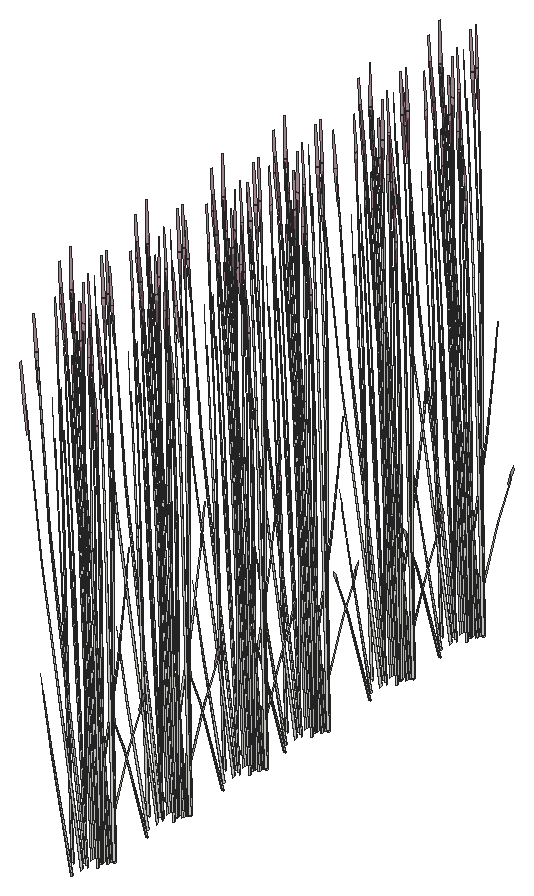
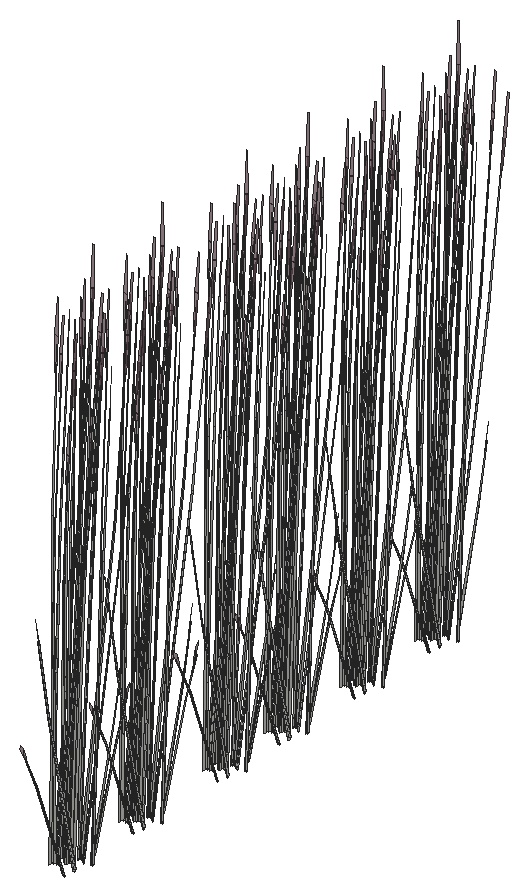
# SketchUp Ruby script. Lengths in inches.
U = 1.inch
M = Sketchup.active_model
def pt(a) = Geom::Point3d.new(a.map { |v| v * U })
def face(e, loops, mat)
  f = e.add_face(loops[0].map { |a| pt(a) })
  loops[1..].each { |l| e.add_face(l.map { |a| pt(a) }).erase! }
  f.material = f.back_material = mat if mat
  f
end
# faces: each face lists its corners as indices into pts; further lists are holes
def faces(e, pts, list, mat = nil) = list.each { |f| face(e, (f[0].is_a?(Array) ? f : [f]).map { |l| l.map { |i| pts[i] } }, mat) }
# xy, xz, yz: faces in a plane at the given z, y or x. An outline is a flat list of corners, or four numbers for a rectangle; further outlines are holes
def ring(l) = l.size == 4 ? [[l[0], l[1]], [l[2], l[1]], [l[2], l[3]], [l[0], l[3]]] : l.each_slice(2).to_a
def flat(e, list, mat, &to3) = list.each { |f| face(e, (f[0].is_a?(Array) ? f : [f]).map { |l| ring(l).map { |u, v| to3.(u, v) } }, mat) }
def xy(e, z, list, mat = nil) = flat(e, list, mat) { |x, y| [x, y, z] }
def xz(e, y, list, mat = nil) = flat(e, list, mat) { |x, z| [x, y, z] }
def yz(e, x, list, mat = nil) = flat(e, list, mat) { |y, z| [x, y, z] }
def lines(e, pts, list) = list.each { |a, b| e.add_line(pt(pts[a]), pt(pts[b])) }
# prism: a flat outline (further loops are holes) pulled along v
def prism(e, loops, v, mat = nil)
  f = face(e, loops, mat); d = Geom::Vector3d.new(v.map { |x| x * U })
  f.pushpull(f.normal.samedirection?(d) ? d.length : -d.length)
end
def box(e, o, s, mat = nil) = prism(e, [[o, [o[0] + s[0], o[1], o[2]], [o[0] + s[0], o[1] + s[1], o[2]], [o[0], o[1] + s[1], o[2]]]], [0, 0, s[2]], mat)
def at(x, y, z, deg = 0) = Geom::Transformation.translation(pt([x, y, z])) * Geom::Transformation.rotation(ORIGIN, Z_AXIS, deg.degrees)
def axes(o, x, y, z) = Geom::Transformation.new([*x, 0, *y, 0, *z, 0, *pt(o).to_a, 1])
def part(name) = M.definitions.add(name)
# library, detail: a bought-in or finely detailed component or shape, given as its bounding box
def library(name, o, s) = part(name).tap { |d| box(d.entities, o, s) }
def detail(e, o, s) = box(e.add_group.entities, o, s)
def put(e, d, t, mat = nil) = e.add_instance(d, t).tap { |i| i.material = mat if mat }
def group(e, t, mat = nil) = e.add_group.tap { |g| g.transformation = t; g.material = mat if mat }.entities
root = M.entities
M.materials.add("LightPink_Translucent").color = [144, 107, 117]
M.materials["LightPink_Translucent"].alpha = 0.75
c1 = part("blade")
p = [[2.15,0.21,22],[0,0.17,0],[0.09,0.45,0],[2.18,0.31,22],[2.29,0.31,22],[0.38,0.45,0],
  [2.48,0.24,33],[2.49,0.24,33],[2.48,0.22,33]]
faces(c1.entities,p,[[0,1,2,3],[4,5,2,3],[6,3,4,7],[8,0,3,6]])
c2 = part("seeds")
p = [[0.3,-0.1,1.38],[-0.01,-0.03,1.59],[-0.01,-0.03,0.03],[0.14,-0.07,-0.07],[0.29,-0.03,3],[0.15,0.01,3.11]]
faces(c2.entities,p,[[0,1,2,3],[1,0,4,5]],"LightPink_Translucent")
c3 = part("blade with seeds")
put(c3.entities,c1,at(0,0,0))
put(c3.entities,c2,axes([2.4,0.25,30.99],[1.5799,-0.05474,1.17369],[-0.12525,1.92788,0.29478],[-0.07173,-0.02425,1.56792]))
put(root,c3,axes([333,451.01,49.85],[-0.20736,-0.4007,-0.61707],[0.59731,-0.14431,-0.16195],[-0.02292,-0.13569,1.36206]))
put(root,c3,axes([333.61,449.38,49.88],[-0.34892,0.22417,-0.0344],[-0.3197,-0.24551,-0.15595],[-0.02251,-0.06957,0.51438]))
put(root,c3,axes([333.32,451.11,49.95],[0.24498,-0.3521,-0.39531],[0.50902,0.16945,0.19025],[0,-0.08116,1.26923]))
put(root,c3,axes([332.02,450.96,49.79],[0.35245,-0.2438,-0.27372],[0.35245,0.2438,0.27372],[0,-0.07853,1.22797]))
put(root,c3,axes([333.25,451.4,50.36],[-0.56863,-0.18645,-0.25709],[0.2738,-0.39352,-0.44182],[-0.01787,-0.09662,1.41118]))
put(root,c3,axes([332.02,451.3125,50.19],[0,0.39075,0.43871],[-0.56491,0,0],[0,-0.089,1.3917]))
put(root,c3,axes([333.42,451.17,50.09],[0.21952,0.43694,0.40429],[-0.62724,0.15194,0.15865],[0.00767,-0.08029,1.40366]))
put(root,c3,axes([333.31,451.51,50.4],[-0.24498,0.3521,0.39531],[-0.50902,-0.16945,-0.19025],[0,-0.08116,1.26923]))
put(root,c3,axes([334.36,451.55,50.03],[-0.46965,-0.33633,-0.05417],[0.46994,-0.33653,0],[-0.0164,-0.01174,1.55135]))
put(root,c3,axes([333.47,451.59,50.09],[0.63817,0.08233,0.40429],[-0.12987,0.46497,0.15865],[-0.09326,-0.0449,1.40366]))
put(root,c3,axes([333.13,452.34,50.1875],[0.54257,-0.10371,0.15589],[0.13397,0.38597,0.31002],[-0.04839,-0.05624,1.41735]))
put(root,c3,axes([333.94,452.25,49.95],[-0.16474,-0.33688,0],[0.47043,-0.11798,0],[0,0,1.36402]))
put(root,c3,axes([334.74,452.36,50.1875],[0.14586,-0.38834,0.15589],[0.53375,0.1099,0.31002],[-0.0922,0.00189,1.41735]))
put(root,c3,axes([333.83,452.4,49.94],[-0.50902,-0.17543,0],[0.24498,-0.36452,0],[0,0,1.43768]))
put(root,c3,axes([334.49,451.67,50.4],[0.54829,-0.02412,0.39531],[0.04958,0.40041,-0.19025],[-0.09816,0.04058,1.26923]))
put(root,c3,axes([334.61,452.79,49.9375],[-0.31175,-0.39292,-0.04544],[0.52815,-0.21836,0.456],[-0.13015,0.03741,1.44584]))
put(root,c3,axes([334.5,451.84,50.3125],[0.37303,0.23477,0.12794],[-0.31115,0.26487,-0.36534],[-0.08661,0.03581,1.11991]))
put(root,c3,axes([334.89,452.57,50.19],[0.47255,-0.19538,0.43871],[0.28245,0.35034,0],[-0.10763,0.0445,1.3917]))
put(root,c3,axes([334.46,452.74,49.79],[-0.47106,-0.09668,-0.27372],[0.11861,-0.34048,0.27372],[-0.09497,0.03926,1.22797]))
put(root,c3,axes([334.38,451.76,50.36],[0.05884,0.44587,-0.25709],[-0.6128,0.02696,-0.44182],[-0.10791,0.05939,1.41118]))
put(root,c3,axes([334.62,452.59,50.06],[0.63212,0.12701,0.27176],[-0.15814,0.45398,-0.32244],[-0.10462,0.05682,1.45692]))
put(root,c3,axes([335,452.84,50.1],[0.31568,0.39156,0],[-0.52815,0.21836,-0.456],[-0.12029,0.04973,1.44655]))
put(root,c3,axes([333.34,452.96,49.32],[0.08172,-0.02126,1.55816],[0.49154,0.11703,-0.23804],[0.01437,0.1319,0.26541]))
put(root,c3,axes([332.21,453.01,50.49],[0.45869,-0.0692,0.0575],[0.10545,0.27878,-0.76259],[-0.02908,0.14112,0.68355]))
put(root,c3,axes([333.7,458.625,49.32],[-0.08469,0.01408,1.55816],[-0.46834,-0.15847,-0.23804],[0.00786,-0.13218,0.26541]))
put(root,c3,axes([333,460.52,49.85],[-0.20736,-0.4007,-0.61707],[0.59731,-0.14431,-0.16195],[-0.02292,-0.13569,1.36206]))
put(root,c3,axes([333.61,458.9,49.88],[-0.34892,0.22417,-0.0344],[-0.3197,-0.24551,-0.15595],[-0.02251,-0.06957,0.51438]))
put(root,c3,axes([333.32,460.625,49.95],[0.24498,-0.3521,-0.39531],[0.50902,0.16945,0.19025],[0,-0.08116,1.26923]))
put(root,c3,axes([332.02,460.47,49.79],[0.35245,-0.2438,-0.27372],[0.35245,0.2438,0.27372],[0,-0.07853,1.22797]))
put(root,c3,axes([333.25,460.92,50.36],[-0.56863,-0.18645,-0.25709],[0.2738,-0.39352,-0.44182],[-0.01787,-0.09662,1.41118]))
put(root,c3,axes([332.02,460.83,50.19],[0,0.39075,0.43871],[-0.56491,0,0],[0,-0.089,1.3917]))
put(root,c3,axes([333.42,460.68,50.09],[0.21952,0.43694,0.40429],[-0.62724,0.15194,0.15865],[0.00767,-0.08029,1.40366]))
put(root,c3,axes([333.31,461.02,50.4],[-0.24498,0.3521,0.39531],[-0.50902,-0.16945,-0.19025],[0,-0.08116,1.26923]))
put(root,c3,axes([334.36,461.07,50.03],[-0.46965,-0.33633,-0.05417],[0.46994,-0.33653,0],[-0.0164,-0.01174,1.55135]))
put(root,c3,axes([333.47,461.11,50.09],[0.63817,0.08233,0.40429],[-0.12987,0.46497,0.15865],[-0.09326,-0.0449,1.40366]))
put(root,c3,axes([333.13,461.85,50.1875],[0.54257,-0.10371,0.15589],[0.13397,0.38597,0.31002],[-0.04839,-0.05624,1.41735]))
put(root,c3,axes([333.94,461.76,49.95],[-0.16474,-0.33688,0],[0.47043,-0.11798,0],[0,0,1.36402]))
put(root,c3,axes([334.74,461.87,50.1875],[0.14586,-0.38834,0.15589],[0.53375,0.1099,0.31002],[-0.0922,0.00189,1.41735]))
put(root,c3,axes([333.83,461.91,49.94],[-0.50902,-0.17543,0],[0.24498,-0.36452,0],[0,0,1.43768]))
put(root,c3,axes([334.49,461.19,50.4],[0.54829,-0.02412,0.39531],[0.04958,0.40041,-0.19025],[-0.09816,0.04058,1.26923]))
put(root,c3,axes([334.61,462.31,49.9375],[-0.31175,-0.39292,-0.04544],[0.52815,-0.21836,0.456],[-0.13015,0.03741,1.44584]))
put(root,c3,axes([334.5,461.36,50.3125],[0.37303,0.23477,0.12794],[-0.31115,0.26487,-0.36534],[-0.08661,0.03581,1.11991]))
put(root,c3,axes([334.89,462.08,50.19],[0.47255,-0.19538,0.43871],[0.28245,0.35034,0],[-0.10763,0.0445,1.3917]))
put(root,c3,axes([334.46,462.26,49.79],[-0.47106,-0.09668,-0.27372],[0.11861,-0.34048,0.27372],[-0.09497,0.03926,1.22797]))
put(root,c3,axes([334.38,461.27,50.36],[0.05884,0.44587,-0.25709],[-0.6128,0.02696,-0.44182],[-0.10791,0.05939,1.41118]))
put(root,c3,axes([334.62,462.11,50.06],[0.63212,0.12701,0.27176],[-0.15814,0.45398,-0.32244],[-0.10462,0.05682,1.45692]))
put(root,c3,axes([335,462.35,50.1],[0.31568,0.39156,0],[-0.52815,0.21836,-0.456],[-0.12029,0.04973,1.44655]))
put(root,c3,axes([333.34,462.47,49.32],[0.08172,-0.02126,1.55816],[0.49154,0.11703,-0.23804],[0.01437,0.1319,0.26541]))
put(root,c3,axes([332.21,462.52,50.49],[0.45869,-0.0692,0.0575],[0.10545,0.27878,-0.76259],[-0.02908,0.14112,0.68355]))
put(root,c3,axes([333.7,468.18,49.32],[-0.08469,0.01408,1.55816],[-0.46834,-0.15847,-0.23804],[0.00786,-0.13218,0.26541]))
put(root,c3,axes([333,470.08,49.85],[-0.20736,-0.4007,-0.61707],[0.59731,-0.14431,-0.16195],[-0.02292,-0.13569,1.36206]))
put(root,c3,axes([333.61,468.45,49.88],[-0.34892,0.22417,-0.0344],[-0.3197,-0.24551,-0.15595],[-0.02251,-0.06957,0.51438]))
put(root,c3,axes([333.32,470.18,49.95],[0.24498,-0.3521,-0.39531],[0.50902,0.16945,0.19025],[0,-0.08116,1.26923]))
put(root,c3,axes([332.02,470.03,49.79],[0.35245,-0.2438,-0.27372],[0.35245,0.2438,0.27372],[0,-0.07853,1.22797]))
put(root,c3,axes([333.25,470.47,50.36],[-0.56863,-0.18645,-0.25709],[0.2738,-0.39352,-0.44182],[-0.01787,-0.09662,1.41118]))
put(root,c3,axes([332.02,470.38,50.19],[0,0.39075,0.43871],[-0.56491,0,0],[0,-0.089,1.3917]))
put(root,c3,axes([333.42,470.24,50.09],[0.21952,0.43694,0.40429],[-0.62724,0.15194,0.15865],[0.00767,-0.08029,1.40366]))
put(root,c3,axes([333.31,470.58,50.4],[-0.24498,0.3521,0.39531],[-0.50902,-0.16945,-0.19025],[0,-0.08116,1.26923]))
put(root,c3,axes([334.36,470.625,50.03],[-0.46965,-0.33633,-0.05417],[0.46994,-0.33653,0],[-0.0164,-0.01174,1.55135]))
put(root,c3,axes([333.47,470.66,50.09],[0.63817,0.08233,0.40429],[-0.12987,0.46497,0.15865],[-0.09326,-0.0449,1.40366]))
put(root,c3,axes([333.13,471.41,50.1875],[0.54257,-0.10371,0.15589],[0.13397,0.38597,0.31002],[-0.04839,-0.05624,1.41735]))
put(root,c3,axes([333.94,471.32,49.95],[-0.16474,-0.33688,0],[0.47043,-0.11798,0],[0,0,1.36402]))
put(root,c3,axes([334.74,471.43,50.1875],[0.14586,-0.38834,0.15589],[0.53375,0.1099,0.31002],[-0.0922,0.00189,1.41735]))
put(root,c3,axes([333.83,471.47,49.94],[-0.50902,-0.17543,0],[0.24498,-0.36452,0],[0,0,1.43768]))
put(root,c3,axes([334.49,470.74,50.4],[0.54829,-0.02412,0.39531],[0.04958,0.40041,-0.19025],[-0.09816,0.04058,1.26923]))
put(root,c3,axes([334.61,471.86,49.9375],[-0.31175,-0.39292,-0.04544],[0.52815,-0.21836,0.456],[-0.13015,0.03741,1.44584]))
put(root,c3,axes([334.5,470.91,50.3125],[0.37303,0.23477,0.12794],[-0.31115,0.26487,-0.36534],[-0.08661,0.03581,1.11991]))
put(root,c3,axes([334.89,471.64,50.19],[0.47255,-0.19538,0.43871],[0.28245,0.35034,0],[-0.10763,0.0445,1.3917]))
put(root,c3,axes([334.46,471.8125,49.79],[-0.47106,-0.09668,-0.27372],[0.11861,-0.34048,0.27372],[-0.09497,0.03926,1.22797]))
put(root,c3,axes([334.38,470.83,50.36],[0.05884,0.44587,-0.25709],[-0.6128,0.02696,-0.44182],[-0.10791,0.05939,1.41118]))
put(root,c3,axes([334.62,471.66,50.06],[0.63212,0.12701,0.27176],[-0.15814,0.45398,-0.32244],[-0.10462,0.05682,1.45692]))
put(root,c3,axes([335,471.91,50.1],[0.31568,0.39156,0],[-0.52815,0.21836,-0.456],[-0.12029,0.04973,1.44655]))
put(root,c3,axes([333.7,475.98,49.32],[-0.08469,0.01408,1.55816],[-0.46834,-0.15847,-0.23804],[0.00786,-0.13218,0.26541]))
put(root,c3,axes([333.34,472.03,49.32],[0.08172,-0.02126,1.55816],[0.49154,0.11703,-0.23804],[0.01437,0.1319,0.26541]))
put(root,c3,axes([332.21,472.08,50.49],[0.45869,-0.0692,0.0575],[0.10545,0.27878,-0.76259],[-0.02908,0.14112,0.68355]))
put(root,c3,axes([333,477.875,49.85],[-0.20736,-0.4007,-0.61707],[0.59731,-0.14431,-0.16195],[-0.02292,-0.13569,1.36206]))
put(root,c3,axes([333.61,476.25,49.88],[-0.34892,0.22417,-0.0344],[-0.3197,-0.24551,-0.15595],[-0.02251,-0.06957,0.51438]))
put(root,c3,axes([333.32,477.98,49.95],[0.24498,-0.3521,-0.39531],[0.50902,0.16945,0.19025],[0,-0.08116,1.26923]))
put(root,c3,axes([332.02,477.83,49.79],[0.35245,-0.2438,-0.27372],[0.35245,0.2438,0.27372],[0,-0.07853,1.22797]))
put(root,c3,axes([333.25,478.27,50.36],[-0.56863,-0.18645,-0.25709],[0.2738,-0.39352,-0.44182],[-0.01787,-0.09662,1.41118]))
put(root,c3,axes([332.02,478.18,50.19],[0,0.39075,0.43871],[-0.56491,0,0],[0,-0.089,1.3917]))
put(root,c3,axes([333.42,478.03,50.09],[0.21952,0.43694,0.40429],[-0.62724,0.15194,0.15865],[0.00767,-0.08029,1.40366]))
put(root,c3,axes([333.31,478.38,50.4],[-0.24498,0.3521,0.39531],[-0.50902,-0.16945,-0.19025],[0,-0.08116,1.26923]))
put(root,c3,axes([334.36,478.42,50.03],[-0.46965,-0.33633,-0.05417],[0.46994,-0.33653,0],[-0.0164,-0.01174,1.55135]))
put(root,c3,axes([333.47,478.46,50.09],[0.63817,0.08233,0.40429],[-0.12987,0.46497,0.15865],[-0.09326,-0.0449,1.40366]))
put(root,c3,axes([333.13,479.2,50.1875],[0.54257,-0.10371,0.15589],[0.13397,0.38597,0.31002],[-0.04839,-0.05624,1.41735]))
put(root,c3,axes([333.94,479.11,49.95],[-0.16474,-0.33688,0],[0.47043,-0.11798,0],[0,0,1.36402]))
put(root,c3,axes([334.74,479.23,50.1875],[0.14586,-0.38834,0.15589],[0.53375,0.1099,0.31002],[-0.0922,0.00189,1.41735]))
put(root,c3,axes([333.83,479.27,49.94],[-0.50902,-0.17543,0],[0.24498,-0.36452,0],[0,0,1.43768]))
put(root,c3,axes([334.49,478.54,50.4],[0.54829,-0.02412,0.39531],[0.04958,0.40041,-0.19025],[-0.09816,0.04058,1.26923]))
put(root,c3,axes([334.61,479.66,49.9375],[-0.31175,-0.39292,-0.04544],[0.52815,-0.21836,0.456],[-0.13015,0.03741,1.44584]))
put(root,c3,axes([334.5,478.71,50.3125],[0.37303,0.23477,0.12794],[-0.31115,0.26487,-0.36534],[-0.08661,0.03581,1.11991]))
put(root,c3,axes([334.89,479.43,50.19],[0.47255,-0.19538,0.43871],[0.28245,0.35034,0],[-0.10763,0.0445,1.3917]))
put(root,c3,axes([334.46,479.61,49.79],[-0.47106,-0.09668,-0.27372],[0.11861,-0.34048,0.27372],[-0.09497,0.03926,1.22797]))
put(root,c3,axes([334.38,478.625,50.36],[0.05884,0.44587,-0.25709],[-0.6128,0.02696,-0.44182],[-0.10791,0.05939,1.41118]))
put(root,c3,axes([334.62,479.46,50.06],[0.63212,0.12701,0.27176],[-0.15814,0.45398,-0.32244],[-0.10462,0.05682,1.45692]))
put(root,c3,axes([335,479.7,50.1],[0.31568,0.39156,0],[-0.52815,0.21836,-0.456],[-0.12029,0.04973,1.44655]))
put(root,c3,axes([333.34,479.82,49.32],[0.08172,-0.02126,1.55816],[0.49154,0.11703,-0.23804],[0.01437,0.1319,0.26541]))
put(root,c3,axes([332.21,479.875,50.49],[0.45869,-0.0692,0.0575],[0.10545,0.27878,-0.76259],[-0.02908,0.14112,0.68355]))
put(root,c3,axes([333.7,486.68,49.32],[-0.08469,0.01408,1.55816],[-0.46834,-0.15847,-0.23804],[0.00786,-0.13218,0.26541]))
put(root,c3,axes([333,488.57,49.85],[-0.20736,-0.4007,-0.61707],[0.59731,-0.14431,-0.16195],[-0.02292,-0.13569,1.36206]))
put(root,c3,axes([333.61,486.95,49.88],[-0.34892,0.22417,-0.0344],[-0.3197,-0.24551,-0.15595],[-0.02251,-0.06957,0.51438]))
put(root,c3,axes([333.32,488.68,49.95],[0.24498,-0.3521,-0.39531],[0.50902,0.16945,0.19025],[0,-0.08116,1.26923]))
put(root,c3,axes([332.02,488.53,49.79],[0.35245,-0.2438,-0.27372],[0.35245,0.2438,0.27372],[0,-0.07853,1.22797]))
put(root,c3,axes([333.25,488.97,50.36],[-0.56863,-0.18645,-0.25709],[0.2738,-0.39352,-0.44182],[-0.01787,-0.09662,1.41118]))
put(root,c3,axes([332.02,488.88,50.19],[0,0.39075,0.43871],[-0.56491,0,0],[0,-0.089,1.3917]))
put(root,c3,axes([333.42,488.73,50.09],[0.21952,0.43694,0.40429],[-0.62724,0.15194,0.15865],[0.00767,-0.08029,1.40366]))
put(root,c3,axes([333.31,489.08,50.4],[-0.24498,0.3521,0.39531],[-0.50902,-0.16945,-0.19025],[0,-0.08116,1.26923]))
put(root,c3,axes([334.36,489.12,50.03],[-0.46965,-0.33633,-0.05417],[0.46994,-0.33653,0],[-0.0164,-0.01174,1.55135]))
put(root,c3,axes([333.47,489.16,50.09],[0.63817,0.08233,0.40429],[-0.12987,0.46497,0.15865],[-0.09326,-0.0449,1.40366]))
put(root,c3,axes([333.13,489.9,50.1875],[0.54257,-0.10371,0.15589],[0.13397,0.38597,0.31002],[-0.04839,-0.05624,1.41735]))
put(root,c3,axes([333.94,489.8125,49.95],[-0.16474,-0.33688,0],[0.47043,-0.11798,0],[0,0,1.36402]))
put(root,c3,axes([334.74,489.93,50.1875],[0.14586,-0.38834,0.15589],[0.53375,0.1099,0.31002],[-0.0922,0.00189,1.41735]))
put(root,c3,axes([333.83,489.97,49.94],[-0.50902,-0.17543,0],[0.24498,-0.36452,0],[0,0,1.43768]))
put(root,c3,axes([334.49,489.24,50.4],[0.54829,-0.02412,0.39531],[0.04958,0.40041,-0.19025],[-0.09816,0.04058,1.26923]))
put(root,c3,axes([334.61,490.36,49.9375],[-0.31175,-0.39292,-0.04544],[0.52815,-0.21836,0.456],[-0.13015,0.03741,1.44584]))
put(root,c3,axes([334.5,489.41,50.3125],[0.37303,0.23477,0.12794],[-0.31115,0.26487,-0.36534],[-0.08661,0.03581,1.11991]))
put(root,c3,axes([334.89,490.13,50.19],[0.47255,-0.19538,0.43871],[0.28245,0.35034,0],[-0.10763,0.0445,1.3917]))
put(root,c3,axes([334.46,490.3125,49.79],[-0.47106,-0.09668,-0.27372],[0.11861,-0.34048,0.27372],[-0.09497,0.03926,1.22797]))
put(root,c3,axes([334.38,489.32,50.36],[0.05884,0.44587,-0.25709],[-0.6128,0.02696,-0.44182],[-0.10791,0.05939,1.41118]))
put(root,c3,axes([334.62,490.16,50.06],[0.63212,0.12701,0.27176],[-0.15814,0.45398,-0.32244],[-0.10462,0.05682,1.45692]))
put(root,c3,axes([335,490.4,50.1],[0.31568,0.39156,0],[-0.52815,0.21836,-0.456],[-0.12029,0.04973,1.44655]))
put(root,c3,axes([333.34,490.52,49.32],[0.08172,-0.02126,1.55816],[0.49154,0.11703,-0.23804],[0.01437,0.1319,0.26541]))
put(root,c3,axes([333.7,495.45,49.32],[-0.08469,0.01408,1.55816],[-0.46834,-0.15847,-0.23804],[0.00786,-0.13218,0.26541]))
put(root,c3,axes([332.21,490.58,50.49],[0.45869,-0.0692,0.0575],[0.10545,0.27878,-0.76259],[-0.02908,0.14112,0.68355]))
put(root,c3,axes([333,497.35,49.85],[-0.20736,-0.4007,-0.61707],[0.59731,-0.14431,-0.16195],[-0.02292,-0.13569,1.36206]))
put(root,c3,axes([333.61,495.73,49.88],[-0.34892,0.22417,-0.0344],[-0.3197,-0.24551,-0.15595],[-0.02251,-0.06957,0.51438]))
put(root,c3,axes([333.32,497.46,49.95],[0.24498,-0.3521,-0.39531],[0.50902,0.16945,0.19025],[0,-0.08116,1.26923]))
put(root,c3,axes([332.02,497.3,49.79],[0.35245,-0.2438,-0.27372],[0.35245,0.2438,0.27372],[0,-0.07853,1.22797]))
put(root,c3,axes([333.25,497.75,50.36],[-0.56863,-0.18645,-0.25709],[0.2738,-0.39352,-0.44182],[-0.01787,-0.09662,1.41118]))
put(root,c3,axes([332.02,497.66,50.19],[0,0.39075,0.43871],[-0.56491,0,0],[0,-0.089,1.3917]))
put(root,c3,axes([333.42,497.51,50.09],[0.21952,0.43694,0.40429],[-0.62724,0.15194,0.15865],[0.00767,-0.08029,1.40366]))
put(root,c3,axes([333.31,497.86,50.4],[-0.24498,0.3521,0.39531],[-0.50902,-0.16945,-0.19025],[0,-0.08116,1.26923]))
put(root,c3,axes([334.36,497.9,50.03],[-0.46965,-0.33633,-0.05417],[0.46994,-0.33653,0],[-0.0164,-0.01174,1.55135]))
put(root,c3,axes([333.47,497.9375,50.09],[0.63817,0.08233,0.40429],[-0.12987,0.46497,0.15865],[-0.09326,-0.0449,1.40366]))
put(root,c3,axes([333.13,498.68,50.1875],[0.54257,-0.10371,0.15589],[0.13397,0.38597,0.31002],[-0.04839,-0.05624,1.41735]))
put(root,c3,axes([333.94,498.59,49.95],[-0.16474,-0.33688,0],[0.47043,-0.11798,0],[0,0,1.36402]))
put(root,c3,axes([334.74,498.7,50.1875],[0.14586,-0.38834,0.15589],[0.53375,0.1099,0.31002],[-0.0922,0.00189,1.41735]))
put(root,c3,axes([333.83,498.74,49.94],[-0.50902,-0.17543,0],[0.24498,-0.36452,0],[0,0,1.43768]))
put(root,c3,axes([334.49,498.02,50.4],[0.54829,-0.02412,0.39531],[0.04958,0.40041,-0.19025],[-0.09816,0.04058,1.26923]))
put(root,c3,axes([334.61,499.14,49.9375],[-0.31175,-0.39292,-0.04544],[0.52815,-0.21836,0.456],[-0.13015,0.03741,1.44584]))
put(root,c3,axes([334.5,498.1875,50.3125],[0.37303,0.23477,0.12794],[-0.31115,0.26487,-0.36534],[-0.08661,0.03581,1.11991]))
put(root,c3,axes([334.89,498.91,50.19],[0.47255,-0.19538,0.43871],[0.28245,0.35034,0],[-0.10763,0.0445,1.3917]))
put(root,c3,axes([334.46,499.09,49.79],[-0.47106,-0.09668,-0.27372],[0.11861,-0.34048,0.27372],[-0.09497,0.03926,1.22797]))
put(root,c3,axes([334.38,498.1,50.36],[0.05884,0.44587,-0.25709],[-0.6128,0.02696,-0.44182],[-0.10791,0.05939,1.41118]))
put(root,c3,axes([334.62,498.9375,50.06],[0.63212,0.12701,0.27176],[-0.15814,0.45398,-0.32244],[-0.10462,0.05682,1.45692]))
put(root,c3,axes([335,499.18,50.1],[0.31568,0.39156,0],[-0.52815,0.21836,-0.456],[-0.12029,0.04973,1.44655]))
put(root,c3,axes([333.34,499.3,49.32],[0.08172,-0.02126,1.55816],[0.49154,0.11703,-0.23804],[0.01437,0.1319,0.26541]))
put(root,c3,axes([332.21,499.35,50.49],[0.45869,-0.0692,0.0575],[0.10545,0.27878,-0.76259],[-0.02908,0.14112,0.68355]))
